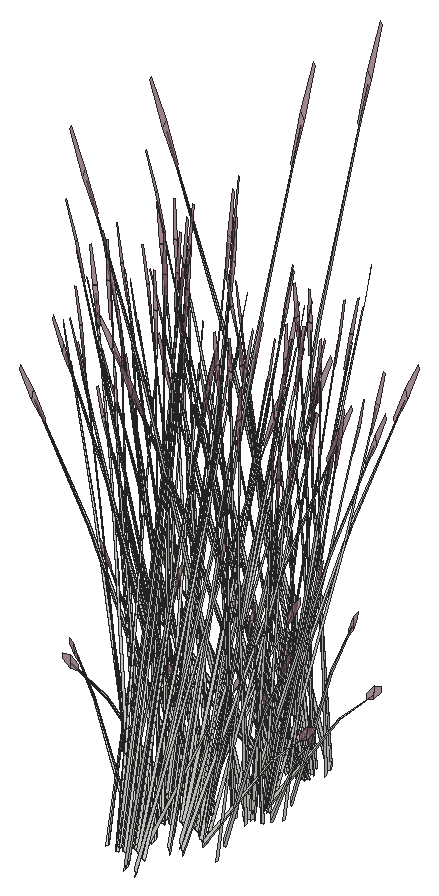
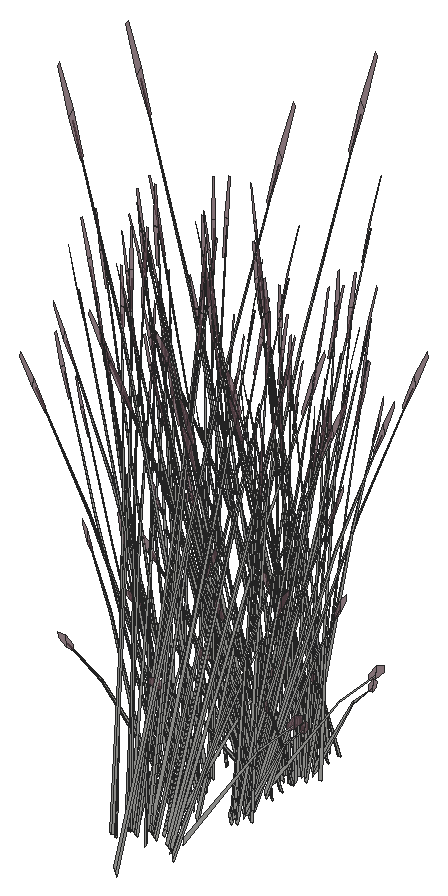
# SketchUp Ruby script. Lengths in inches.
U = 1.inch
M = Sketchup.active_model
def pt(a) = Geom::Point3d.new(a.map { |v| v * U })
def face(e, loops, mat)
  f = e.add_face(loops[0].map { |a| pt(a) })
  loops[1..].each { |l| e.add_face(l.map { |a| pt(a) }).erase! }
  f.material = f.back_material = mat if mat
  f
end
# faces: each face lists its corners as indices into pts; further lists are holes
def faces(e, pts, list, mat = nil) = list.each { |f| face(e, (f[0].is_a?(Array) ? f : [f]).map { |l| l.map { |i| pts[i] } }, mat) }
# xy, xz, yz: faces in a plane at the given z, y or x. An outline is a flat list of corners, or four numbers for a rectangle; further outlines are holes
def ring(l) = l.size == 4 ? [[l[0], l[1]], [l[2], l[1]], [l[2], l[3]], [l[0], l[3]]] : l.each_slice(2).to_a
def flat(e, list, mat, &to3) = list.each { |f| face(e, (f[0].is_a?(Array) ? f : [f]).map { |l| ring(l).map { |u, v| to3.(u, v) } }, mat) }
def xy(e, z, list, mat = nil) = flat(e, list, mat) { |x, y| [x, y, z] }
def xz(e, y, list, mat = nil) = flat(e, list, mat) { |x, z| [x, y, z] }
def yz(e, x, list, mat = nil) = flat(e, list, mat) { |y, z| [x, y, z] }
def lines(e, pts, list) = list.each { |a, b| e.add_line(pt(pts[a]), pt(pts[b])) }
# prism: a flat outline (further loops are holes) pulled along v
def prism(e, loops, v, mat = nil)
  f = face(e, loops, mat); d = Geom::Vector3d.new(v.map { |x| x * U })
  f.pushpull(f.normal.samedirection?(d) ? d.length : -d.length)
end
def box(e, o, s, mat = nil) = prism(e, [[o, [o[0] + s[0], o[1], o[2]], [o[0] + s[0], o[1] + s[1], o[2]], [o[0], o[1] + s[1], o[2]]]], [0, 0, s[2]], mat)
def at(x, y, z, deg = 0) = Geom::Transformation.translation(pt([x, y, z])) * Geom::Transformation.rotation(ORIGIN, Z_AXIS, deg.degrees)
def axes(o, x, y, z) = Geom::Transformation.new([*x, 0, *y, 0, *z, 0, *pt(o).to_a, 1])
def part(name) = M.definitions.add(name)
# library, detail: a bought-in or finely detailed component or shape, given as its bounding box
def library(name, o, s) = part(name).tap { |d| box(d.entities, o, s) }
def detail(e, o, s) = box(e.add_group.entities, o, s)
def put(e, d, t, mat = nil) = e.add_instance(d, t).tap { |i| i.material = mat if mat }
def group(e, t, mat = nil) = e.add_group.tap { |g| g.transformation = t; g.material = mat if mat }.entities
root = M.entities
M.materials.add("LightPink_Translucent").color = [144, 107, 117]
M.materials["LightPink_Translucent"].alpha = 0.75
c1 = part("blade")
p = [[2.15,0.21,22],[0,0.17,0],[0.09,0.45,0],[2.18,0.31,22],[2.29,0.31,22],[0.38,0.45,0],
  [2.48,0.24,33],[2.49,0.24,33],[2.48,0.22,33]]
faces(c1.entities,p,[[0,1,2,3],[4,5,2,3],[6,3,4,7],[8,0,3,6]])
c2 = part("seeds")
p = [[0.3,-0.1,1.38],[-0.01,-0.03,1.59],[-0.01,-0.03,0.03],[0.14,-0.07,-0.07],[0.29,-0.03,3],[0.15,0.01,3.11]]
faces(c2.entities,p,[[0,1,2,3],[1,0,4,5]],"LightPink_Translucent")
c3 = part("blade with seeds")
put(c3.entities,c1,at(0,0,0))
put(c3.entities,c2,axes([2.4,0.25,30.99],[1.5799,-0.05474,1.17369],[-0.12525,1.92788,0.29478],[-0.07173,-0.02425,1.56792]))
put(root,c3,axes([428.66,442.95,154],[-0.30197,0.1603,0.05432],[-0.1478,-0.29231,0.42765],[0.02916,0.12885,0.65209]))
put(root,c3,axes([427.85,442.5625,153.82],[-0.27728,0.24833,-0.29918],[-0.26248,-0.28355,0.38624],[-0.03994,0.14407,0.73904]))
put(root,c3,axes([426.9,442.49,153.98],[-0.01019,0.09334,1.47793],[0.28908,0.3247,-0.23373],[-0.07568,0.15355,0.11853]))
put(root,c3,axes([427.82,442.28,154.56],[0.45039,0.02337,-0.11403],[-0.01231,0.44247,-0.63292],[-0.03129,0.17041,0.9617]))
put(root,c3,axes([428.66,442.77,154.25],[0.40102,-0.2196,-0.10273],[0.19707,0.38974,-0.57019],[0.05291,0.16424,0.8664]))
put(root,c3,axes([431.71,446.31,153.98],[-0.03706,-0.04129,1.49853],[0.08106,-0.44261,-0.1416],[0.14596,-0.02828,0.26519]))
put(root,c3,axes([426.89,444.51,153.98],[-0.06692,0.06124,1.47793],[0.00569,0.44742,-0.23373],[-0.15339,0.05818,0.11853]))
put(root,c3,axes([427.34,444.45,153.95],[-0.11102,0.42903,-0.43168],[-0.38064,-0.14706,-0.33437],[-0.15325,0.03934,0.82598]))
put(root,c3,axes([427.32,444.08,154.25],[0.20619,0.42709,-0.10273],[-0.36595,0.20988,-0.57019],[-0.15422,0.05635,0.8664]))
put(root,c3,axes([431.39,445.9375,153.32],[-0.07843,-0.39649,-0.0295],[0.37072,-0.09115,-0.13375],[0.07742,0.02514,0.44114]))
put(root,c3,axes([428.51,447.95,154],[0.18625,-0.29962,0.05432],[0.26523,0.17444,0.42765],[-0.08575,-0.09606,0.65209]))
put(root,c3,axes([430.43,445.93,154.25],[0.02194,-0.47967,-0.10273],[0.41546,0.01311,-0.57019],[0.16001,0.03332,0.8664]))
put(root,c3,axes([428.13,442.45,154.23],[0.29336,0.31691,-0.47917],[-0.3099,0.27755,-0.37115],[-0.04464,0.16102,0.91684]))
put(root,c3,axes([427.57,448.54,153.27],[0.15222,0.08126,1.44779],[-0.31502,0.34091,0.11706],[-0.19634,-0.15379,0.61892]))
put(root,c3,axes([429,442.75,153.95],[0.40284,0.11824,-0.43168],[-0.13808,0.40538,-0.33437],[0.03694,0.16321,0.82598]))
put(root,c3,axes([429.23,441.92,153.27],[-0.09368,-0.15143,1.44779],[0.43286,-0.12749,0.11706],[0.09783,0.23774,0.61892]))
put(root,c3,axes([428.82,443,153.82],[-0.12355,0.36271,-0.29918],[-0.36044,-0.10579,0.38624],[0.03305,0.14603,0.73904]))
put(root,c3,axes([428.31,448.3,153.95],[-0.40438,0.11212,-0.43168],[-0.07074,-0.4246,-0.33437],[-0.10862,-0.12168,0.82598]))
put(root,c3,axes([430.35,448.39,154],[0.29182,0.32181,0.40553],[-0.3099,0.27755,0.33437],[0.05383,-0.15098,0.83914]))
put(root,c3,axes([428.59,447.92,154.59],[-0.2735,0.45217,-0.11506],[-0.39608,-0.2605,-0.63862],[-0.13768,-0.12775,0.97037]))
put(root,c3,axes([430.46,448.42,154],[0.33677,0.02198,0.05432],[-0.00923,0.33185,0.42765],[0.03524,-0.12712,0.65209]))
put(root,c3,axes([428.04,442.3,154.51],[-0.01066,0.43628,-0.66621],[-0.44902,-0.0293,0.0804],[-0.04739,0.18483,0.94242]))
put(root,c3,axes([426.87,443.45,153.98],[0.04649,-0.02848,1.49853],[0.38427,0.18941,-0.1416],[-0.00903,0.15771,0.26519]))
put(root,c3,axes([430.6875,449.14,153.95],[-0.10528,-0.43067,-0.43168],[0.39868,-0.07534,-0.33437],[0.11425,-0.11568,0.82598]))
put(root,c3,axes([428.46,441.99,153.27],[-0.01003,-0.18103,1.44779],[0.43473,0.12009,0.11706],[-0.02689,0.25798,0.61892]))
put(root,c3,axes([430.79,445.64,153.98],[0.08791,-0.00798,1.47793],[0.24113,-0.36643,-0.23373],[0.15637,0.04837,0.11853]))
put(root,c3,axes([427.27,445.28,154],[-0.10163,-0.43409,0.40553],[0.39868,-0.07534,0.33437],[-0.1175,0.10209,0.83914]))
put(root,c3,axes([427.19,445.2,154],[-0.28133,-0.19836,0.05432],[0.16379,-0.28248,0.42765],[-0.0902,0.09132,0.65209]))
put(root,c3,axes([427.32,444.67,153.27],[0.14219,-0.09977,1.44779],[0.11971,0.461,0.11706],[-0.22323,0.10419,0.61892]))
put(root,c3,axes([427.54,447.79,153.98],[-0.08817,-0.00333,1.47793],[-0.28072,0.33293,-0.23373],[-0.14978,-0.06803,0.11853]))
put(root,c3,axes([430.875,449.45,154.25],[-0.37908,-0.26007,-0.10273],[0.21839,-0.37663,-0.57019],[0.1071,-0.13092,0.8664]))
put(root,c3,axes([428.5625,443.64,153.98],[0.05195,0.07595,1.47793],[0.41921,0.02984,-0.23373],[0.04216,0.1675,0.11853]))
put(root,c3,axes([429.31,450.87,152.81],[0.35414,0.19019,1.27785],[-0.34693,0.40974,0.50532],[-0.1554,-0.24285,1.07126]))
put(root,c3,axes([431.81,449.33,153.98],[-0.05353,-0.00358,1.49853],[-0.22227,-0.38383,-0.1416],[0.08926,-0.1262,0.26519]))
put(root,c3,axes([426.14,444.96,153.98],[0.0523,0.01265,1.49853],[0.16179,0.41674,-0.1416],[-0.10706,0.10938,0.26519]))
put(root,c3,axes([430.69,445.89,153.82],[0.23317,0.29531,-0.29918],[-0.26625,0.27955,0.38624],[0.13527,0.04253,0.73904]))
put(root,c3,axes([430.57,446.01,154],[-0.02064,0.35866,0.05432],[-0.3116,-0.00983,0.42765],[0.11936,0.03753,0.65209]))
put(root,c3,axes([427.23,445.36,153.82],[-0.35672,0.06741,-0.29918],[-0.09419,-0.38534,0.38624],[-0.10222,0.1035,0.73904]))
put(root,c3,axes([427.89,442.92,152.84],[0.009,-0.24349,1.30391],[0.40497,0.12861,0.18019],[-0.03509,0.2595,0.61571]))
put(root,c3,axes([430.98,449.18,153.82],[0.35672,-0.06741,-0.29918],[0.09419,0.38534,0.38624],[0.10222,-0.1035,0.73904]))
put(root,c3,axes([430.6,445.89,154],[-0.30217,0.31079,0.40553],[-0.2606,-0.33005,0.33437],[0.14177,0.05733,0.83914]))
put(root,c3,axes([427.63,448.54,154],[0.02064,-0.35866,0.05432],[0.3116,0.00983,0.42765],[-0.11936,-0.03753,0.65209]))
put(root,c3,axes([427.51,448.65,153.82],[-0.23317,-0.29531,-0.29918],[0.26625,-0.27955,0.38624],[-0.13527,-0.04253,0.73904]))
put(root,c3,axes([429.86,445.14,153.27],[-0.15222,-0.08126,1.44779],[0.31502,-0.34091,0.11706],[0.19634,0.15379,0.61892]))
put(root,c3,axes([429.88,444.07,153.78],[-0.35411,-0.24507,1.16821],[0.37391,-0.38156,0.50405],[0.11425,0.22994,1.12919]))
put(root,c3,axes([427.33,445.1,154.25],[0.37908,0.26007,-0.10273],[-0.21839,0.37663,-0.57019],[-0.1071,0.13092,0.8664]))
put(root,c3,axes([429.61,446.45,154.25],[0.2442,-0.40372,-0.10273],[0.35364,0.23259,-0.57019],[0.12293,0.11406,0.8664]))
put(root,c3,axes([431.01,449.35,154],[0.28133,0.19836,0.05432],[-0.16379,0.28248,0.42765],[0.0902,-0.09132,0.65209]))
put(root,c3,axes([430.93,449.27,154],[0.10163,0.43409,0.40553],[-0.39868,0.07534,0.33437],[0.1175,-0.10209,0.83914]))
put(root,c3,axes([427.84,444.98,153.27],[0.10236,-0.14492,1.44779],[0.25844,0.39118,0.11706],[-0.17726,0.17814,0.61892]))
put(root,c3,axes([432.01,449.79,153.98],[0.05687,-0.07184,1.47793],[-0.07279,-0.44069,-0.23373],[0.14268,-0.08356,0.11853]))
put(root,c3,axes([427.52,445.41,153.95],[0.10528,0.43067,-0.43168],[-0.39868,0.07534,-0.33437],[-0.11425,0.11568,0.82598]))
put(root,c3,axes([429.29,446.78,153.98],[0.00121,-0.0571,1.49853],[0.35119,-0.25193,-0.1416],[0.12199,0.08992,0.26519]))
put(root,c3,axes([427.2,448.07,153.98],[0.03038,0.04707,1.49853],[-0.14646,0.42312,-0.1416],[-0.14833,0.00306,0.26519]))
put(root,c3,axes([427.75,446.13,154],[-0.33677,-0.02198,0.05432],[0.00923,-0.33185,0.42765],[-0.03524,0.12712,0.65209]))
put(root,c3,axes([427.85,446.16,154],[-0.29182,-0.32181,0.40553],[0.3099,-0.27755,0.33437],[-0.05383,0.15098,0.83914]))
put(root,c3,axes([429.9,446.25,153.95],[0.40438,-0.11212,-0.43168],[0.07074,0.4246,-0.33437],[0.10862,0.12168,0.82598]))
put(root,c3,axes([427.625,448.95,153.95],[-0.29757,0.31243,-0.43168],[-0.2606,-0.33005,-0.33437],[-0.15119,-0.04754,0.82598]))
put(root,c3,axes([427.78,448.62,154.25],[-0.02194,0.47967,-0.10273],[-0.41546,-0.01311,-0.57019],[-0.16001,-0.03332,0.8664]))
put(root,c3,axes([429.7,446.59,154],[-0.18625,0.29962,0.05432],[-0.26523,-0.17444,0.42765],[0.08575,0.09606,0.65209]))
put(root,c3,axes([430.89,450.46,154.25],[-0.20619,-0.42709,-0.10273],[0.36595,-0.20988,-0.57019],[0.15422,-0.05635,0.8664]))
put(root,c3,axes([430.87,450.09,153.95],[0.11102,-0.42903,-0.43168],[0.38064,0.14706,-0.33437],[0.15325,-0.03934,0.82598]))
put(root,c3,axes([427.25,449.28,153.27],[0.16998,-0.01068,1.44779],[-0.11276,0.46299,0.11706],[-0.24224,-0.02864,0.61892]))
put(root,c3,axes([429.78,446.51,154],[-0.4076,0.10824,0.40553],[-0.07074,-0.4246,0.33437],[0.09586,0.12514,0.83914]))
put(root,c3,axes([427.77,445.34,153.27],[0.0763,-0.16212,1.44779],[0.3201,0.3355,0.11706],[-0.1444,0.2091,0.61892]))
put(root,c3,axes([428.66,446.64,154],[-0.30197,0.1603,0.05432],[-0.1478,-0.29231,0.42765],[0.02916,0.12885,0.65209]))
put(root,c3,axes([427.85,446.25,153.82],[-0.27728,0.24833,-0.29918],[-0.26248,-0.28355,0.38624],[-0.03994,0.14407,0.73904]))
put(root,c3,axes([426.9,446.18,153.98],[-0.01019,0.09334,1.47793],[0.28908,0.3247,-0.23373],[-0.07568,0.15355,0.11853]))
put(root,c3,axes([427.82,445.97,154.56],[0.45039,0.02337,-0.11403],[-0.01231,0.44247,-0.63292],[-0.03129,0.17041,0.9617]))
put(root,c3,axes([428.66,446.46,154.25],[0.40102,-0.2196,-0.10273],[0.19707,0.38974,-0.57019],[0.05291,0.16424,0.8664]))
put(root,c3,axes([427.18,449.63,154],[0.11578,-0.43006,0.40553],[0.38064,0.14706,0.33437],[-0.14969,0.02584,0.83914]))
put(root,c3,axes([428.13,446.14,154.23],[0.29336,0.31691,-0.47917],[-0.3099,0.27755,-0.37115],[-0.04464,0.16102,0.91684]))
put(root,c3,axes([427.15,449.52,154],[-0.15051,-0.3216,0.05432],[0.27447,-0.15741,0.42765],[-0.12099,0.03106,0.65209]))
put(root,c3,axes([429,446.44,153.95],[0.40284,0.11824,-0.43168],[-0.13808,0.40538,-0.33437],[0.03694,0.16321,0.82598]))
put(root,c3,axes([429.23,445.61,153.27],[-0.09368,-0.15143,1.44779],[0.43286,-0.12749,0.11706],[0.09783,0.23774,0.61892]))
put(root,c3,axes([428.82,446.69,153.82],[-0.12355,0.36271,-0.29918],[-0.36044,-0.10579,0.38624],[0.03305,0.14603,0.73904]))
put(root,c3,axes([431.1,450.29,153.82],[0.34057,0.13158,-0.29918],[-0.09933,0.38387,0.38624],[0.13712,-0.0352,0.73904]))
put(root,c3,axes([428.04,445.99,154.51],[-0.01066,0.43628,-0.66621],[-0.44902,-0.0293,0.0804],[-0.04739,0.18483,0.94242]))
put(root,c3,axes([426.87,447.14,153.98],[0.04649,-0.02848,1.49853],[0.38427,0.18941,-0.1416],[-0.00903,0.15771,0.26519]))
put(root,c3,axes([427.1,449.68,153.82],[-0.34057,-0.13158,-0.29918],[0.09933,-0.38387,0.38624],[-0.13712,0.0352,0.73904]))
put(root,c3,axes([428.46,445.68,153.27],[-0.01003,-0.18103,1.44779],[0.43473,0.12009,0.11706],[-0.02689,0.25798,0.61892]))
put(root,c3,axes([430.18,449.8125,153.27],[-0.16998,0.01068,1.44779],[0.11276,-0.46299,0.11706],[0.24224,0.02864,0.61892]))
put(root,c3,axes([431.05,450.45,154],[0.15051,0.3216,0.05432],[-0.27447,0.15741,0.42765],[0.12099,-0.03106,0.65209]))
put(root,c3,axes([431.03,450.34,154],[-0.11578,0.43006,0.40553],[-0.38064,-0.14706,0.33437],[0.14969,-0.02584,0.83914]))
put(root,c3,axes([428.5625,447.34,153.98],[0.05195,0.07595,1.47793],[0.41921,0.02984,-0.23373],[0.04216,0.1675,0.11853]))
put(root,c3,axes([428.2,454.55,153.27],[0.09368,0.15143,1.44779],[-0.43286,0.12749,0.11706],[-0.09783,-0.23774,0.61892]))
put(root,c3,axes([428.91,453.54,153.98],[-0.06268,-0.06613,1.47793],[-0.4183,0.04193,-0.23373],[-0.06676,-0.15817,0.11853]))
put(root,c3,axes([428.14,449.61,152.82],[0.11649,-0.06823,1.49584],[0.04017,0.47639,0.11706],[-0.25231,0.06321,0.53462]))
put(root,c3,axes([427.89,446.61,152.84],[0.009,-0.24349,1.30391],[0.40497,0.12861,0.18019],[-0.03509,0.2595,0.61571]))
put(root,c3,axes([431.71,451.73,153.98],[-0.03706,-0.04129,1.49853],[0.08106,-0.44261,-0.1416],[0.14596,-0.02828,0.26519]))
put(root,c3,axes([426.89,449.93,153.98],[-0.06692,0.06124,1.47793],[0.00569,0.44742,-0.23373],[-0.15339,0.05818,0.11853]))
put(root,c3,axes([427.34,449.875,153.95],[-0.11102,0.42903,-0.43168],[-0.38064,-0.14706,-0.33437],[-0.15325,0.03934,0.82598]))
put(root,c3,axes([430.79,454.35,153.98],[-0.00396,-0.09387,1.47793],[-0.33411,-0.2713,-0.23373],[0.05166,-0.16446,0.11853]))
put(root,c3,axes([427.32,449.51,154.25],[0.20619,0.42709,-0.10273],[-0.36595,0.20988,-0.57019],[-0.15422,0.05635,0.8664]))
put(root,c3,axes([429.39,454.33,153.82],[0.12355,-0.36271,-0.29918],[0.36044,0.10579,0.38624],[-0.03305,-0.14603,0.73904]))
put(root,c3,axes([429.66,454.8125,153.27],[-0.0763,0.16212,1.44779],[-0.3201,-0.3355,0.11706],[0.1444,-0.2091,0.61892]))
put(root,c3,axes([430.7,454.02,153.98],[-0.04162,0.03603,1.49853],[-0.40776,-0.12155,-0.1416],[-0.01476,-0.15722,0.26519]))
put(root,c3,axes([431.39,451.36,153.32],[-0.07843,-0.39649,-0.0295],[0.37072,-0.09115,-0.13375],[0.07742,0.02514,0.44114]))
put(root,c3,axes([430.43,451.35,154.25],[0.02194,-0.47967,-0.10273],[0.41546,0.01311,-0.57019],[0.16001,0.03332,0.8664]))
put(root,c3,axes([429.21,454.58,153.95],[-0.40284,-0.11824,-0.43168],[0.13808,-0.40538,-0.33437],[-0.03694,-0.16321,0.82598]))
put(root,c3,axes([430.08,454.89,153.95],[-0.29336,-0.31691,-0.43168],[0.3099,-0.27755,-0.33437],[0.04464,-0.16102,0.82598]))
put(root,c3,axes([428.49,453.33,153.98],[-0.00765,0.05653,1.49853],[-0.37706,0.20517,-0.1416],[-0.11096,-0.10488,0.26519]))
put(root,c3,axes([429.43,454.42,154],[0.4038,0.12331,0.40553],[-0.13808,0.40538,0.33437],[-0.02427,-0.15942,0.83914]))
put(root,c3,axes([429.55,454.5625,154.25],[-0.40102,0.2196,-0.10273],[-0.19707,-0.38974,-0.57019],[-0.05291,-0.16424,0.8664]))
put(root,c3,axes([430.38,455.06,154.25],[-0.45039,-0.02337,-0.10273],[0.01231,-0.44247,-0.57019],[0.03129,-0.17041,0.8664]))
put(root,c3,axes([430.79,451.06,153.98],[0.08791,-0.00798,1.47793],[0.24113,-0.36643,-0.23373],[0.15637,0.04837,0.11853]))
put(root,c3,axes([430.35,454.77,153.82],[0.27728,-0.24833,-0.29918],[0.26248,0.28355,0.38624],[0.03994,-0.14407,0.73904]))
put(root,c3,axes([429.54,454.39,154],[0.30197,-0.1603,0.05432],[0.1478,0.29231,0.42765],[-0.02916,-0.12885,0.65209]))
put(root,c3,axes([427.27,450.7,154],[-0.10163,-0.43409,0.40553],[0.39868,-0.07534,0.33437],[-0.1175,0.10209,0.83914]))
put(root,c3,axes([427.19,450.62,154],[-0.28133,-0.19836,0.05432],[0.16379,-0.28248,0.42765],[-0.0902,0.09132,0.65209]))
put(root,c3,axes([428.35,454.47,153.82],[-0.06329,-0.37991,-0.29918],[0.36182,-0.10032,0.38624],[-0.09718,-0.10887,0.73904]))
put(root,c3,axes([427.32,450.09,153.27],[0.14219,-0.09977,1.44779],[0.11971,0.461,0.11706],[-0.22323,0.10419,0.61892]))
put(root,c3,axes([428.51,454.43,154],[0.18625,-0.29962,0.05432],[0.26523,0.17444,0.42765],[-0.08575,-0.09606,0.65209]))
put(root,c3,axes([427.57,455.02,153.27],[0.15222,0.08126,1.44779],[-0.31502,0.34091,0.11706],[-0.19634,-0.15379,0.61892]))
put(root,c3,axes([426.14,450.39,153.98],[0.0523,0.01265,1.49853],[0.16179,0.41674,-0.1416],[-0.10706,0.10938,0.26519]))
put(root,c3,axes([430.69,451.3125,153.82],[0.23317,0.29531,-0.29918],[-0.26625,0.27955,0.38624],[0.13527,0.04253,0.73904]))
put(root,c3,axes([430.57,451.43,154],[-0.02064,0.35866,0.05432],[-0.3116,-0.00983,0.42765],[0.11936,0.03753,0.65209]))
put(root,c3,axes([428.31,454.78,153.95],[-0.40438,0.11212,-0.43168],[-0.07074,-0.4246,-0.33437],[-0.10862,-0.12168,0.82598]))
put(root,c3,axes([430.35,454.87,154],[0.29182,0.32181,0.40553],[-0.3099,0.27755,0.33437],[0.05383,-0.15098,0.83914]))
put(root,c3,axes([427.23,450.78,153.82],[-0.35672,0.06741,-0.29918],[-0.09419,-0.38534,0.38624],[-0.10222,0.1035,0.73904]))
put(root,c3,axes([428.59,454.4,154.59],[-0.2735,0.45217,-0.11506],[-0.39608,-0.2605,-0.63862],[-0.13768,-0.12775,0.97037]))
put(root,c3,axes([430.46,454.9,154],[0.33677,0.02198,0.05432],[-0.00923,0.33185,0.42765],[0.03524,-0.12712,0.65209]))
put(root,c3,axes([430.6,451.3125,154],[-0.30217,0.31079,0.40553],[-0.2606,-0.33005,0.33437],[0.14177,0.05733,0.83914]))
put(root,c3,axes([430.6875,455.62,153.95],[-0.10528,-0.43067,-0.43168],[0.39868,-0.07534,-0.33437],[0.11425,-0.11568,0.82598]))
put(root,c3,axes([427.54,454.27,153.98],[-0.08817,-0.00333,1.47793],[-0.28072,0.33293,-0.23373],[-0.14978,-0.06803,0.11853]))
put(root,c3,axes([430.875,455.93,154.25],[-0.37908,-0.26007,-0.10273],[0.21839,-0.37663,-0.57019],[0.1071,-0.13092,0.8664]))
put(root,c3,axes([429.86,450.56,153.27],[-0.15222,-0.08126,1.44779],[0.31502,-0.34091,0.11706],[0.19634,0.15379,0.61892]))
put(root,c3,axes([429.88,449.49,153.78],[-0.35411,-0.24507,1.16821],[0.37391,-0.38156,0.50405],[0.11425,0.22994,1.12919]))
put(root,c3,axes([429.31,457.35,152.81],[0.35414,0.19019,1.27785],[-0.34693,0.40974,0.50532],[-0.1554,-0.24285,1.07126]))
